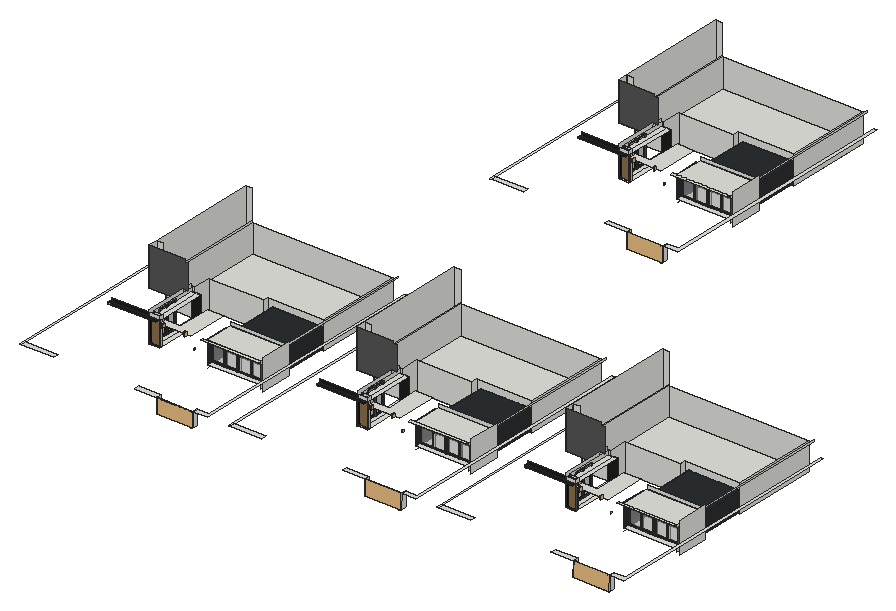
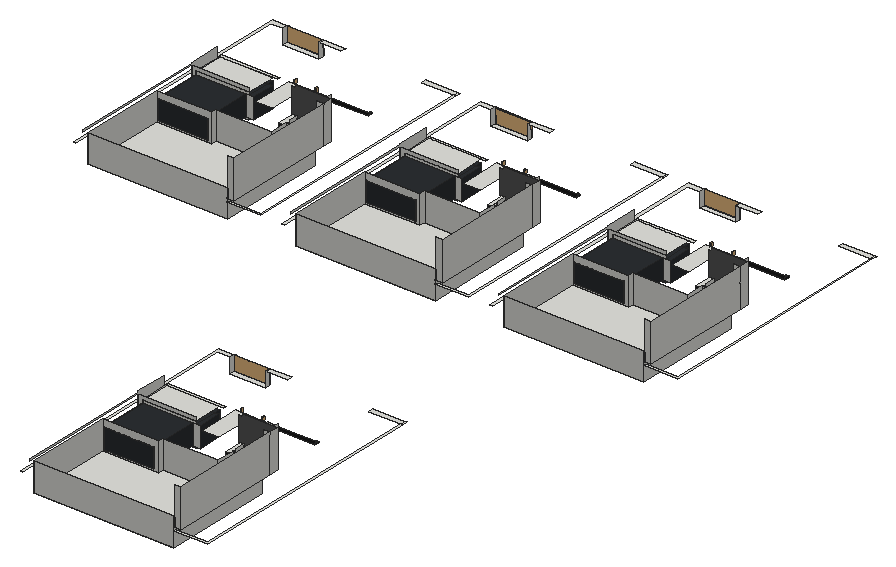
# SketchUp Ruby script. Lengths in inches.
U = 1.inch
M = Sketchup.active_model
def pt(a) = Geom::Point3d.new(a.map { |v| v * U })
def face(e, loops, mat)
  f = e.add_face(loops[0].map { |a| pt(a) })
  loops[1..].each { |l| e.add_face(l.map { |a| pt(a) }).erase! }
  f.material = f.back_material = mat if mat
  f
end
# faces: each face lists its corners as indices into pts; further lists are holes
def faces(e, pts, list, mat = nil) = list.each { |f| face(e, (f[0].is_a?(Array) ? f : [f]).map { |l| l.map { |i| pts[i] } }, mat) }
# xy, xz, yz: faces in a plane at the given z, y or x. An outline is a flat list of corners, or four numbers for a rectangle; further outlines are holes
def ring(l) = l.size == 4 ? [[l[0], l[1]], [l[2], l[1]], [l[2], l[3]], [l[0], l[3]]] : l.each_slice(2).to_a
def flat(e, list, mat, &to3) = list.each { |f| face(e, (f[0].is_a?(Array) ? f : [f]).map { |l| ring(l).map { |u, v| to3.(u, v) } }, mat) }
def xy(e, z, list, mat = nil) = flat(e, list, mat) { |x, y| [x, y, z] }
def xz(e, y, list, mat = nil) = flat(e, list, mat) { |x, z| [x, y, z] }
def yz(e, x, list, mat = nil) = flat(e, list, mat) { |y, z| [x, y, z] }
def lines(e, pts, list) = list.each { |a, b| e.add_line(pt(pts[a]), pt(pts[b])) }
# prism: a flat outline (further loops are holes) pulled along v
def prism(e, loops, v, mat = nil)
  f = face(e, loops, mat); d = Geom::Vector3d.new(v.map { |x| x * U })
  f.pushpull(f.normal.samedirection?(d) ? d.length : -d.length)
end
def box(e, o, s, mat = nil) = prism(e, [[o, [o[0] + s[0], o[1], o[2]], [o[0] + s[0], o[1] + s[1], o[2]], [o[0], o[1] + s[1], o[2]]]], [0, 0, s[2]], mat)
def at(x, y, z, deg = 0) = Geom::Transformation.translation(pt([x, y, z])) * Geom::Transformation.rotation(ORIGIN, Z_AXIS, deg.degrees)
def axes(o, x, y, z) = Geom::Transformation.new([*x, 0, *y, 0, *z, 0, *pt(o).to_a, 1])
def part(name) = M.definitions.add(name)
# library, detail: a bought-in or finely detailed component or shape, given as its bounding box
def library(name, o, s) = part(name).tap { |d| box(d.entities, o, s) }
def detail(e, o, s) = box(e.add_group.entities, o, s)
def put(e, d, t, mat = nil) = e.add_instance(d, t).tap { |i| i.material = mat if mat }
def group(e, t, mat = nil) = e.add_group.tap { |g| g.transformation = t; g.material = mat if mat }.entities
root = M.entities
M.materials.add("Antracyt").color = [44, 47, 50]
M.materials.add("Glass_Tinted_Gray").color = [0, 0, 0]
M.materials["Glass_Tinted_Gray"].alpha = 0.125
M.materials.add("[0135_DarkGray]").color = [81, 81, 81]
M.materials.add("[Color M00]").color = [255, 255, 255]
M.materials.add("[Color M04]").color = [60, 133, 34]
M.materials.add("[Color M06]1").color = [86, 86, 86]
M.materials.add("[Color M08]").color = [30, 30, 30]
M.materials.add("[Mirror 02]").color = [229, 229, 229]
M.materials.add("[Translucent Glass Gray]2").color = [201, 201, 201]
M.materials["[Translucent Glass Gray]2"].alpha = 0.5
M.materials.add("oak swatch").color = [40, 31, 19]
c1 = library("Group\#1",[0,0,0],[29.75,5.78,110.95])
c2 = part("PENTEK_RP Fineline 50S_SlidingDoor_Glass")
box(c2.entities,[0,0,0],[46.58,0.16,94.39],"Glass_Tinted_Gray")
c3 = part("PENTEK_RP Fineline 50S_SlidingDoor_GlazingBead")
box(c3.entities,[0,0,0],[45.47,0.59,0.56],"[0135_DarkGray]")
c4 = part("PENTEK_RP Fineline 50S_SlidingDoor_GlazingBead_2")
box(c4.entities,[0,0,0],[0.56,0.59,94.39],"[0135_DarkGray]")
c5 = part("PENTEK_RP Fineline 50S_SlidingDoor_Leaf_E1")
xy(c5.entities,0,[[0,0,0.93,1.97],[0.93,1.57,1.49,1.97]],"[0135_DarkGray]")
xy(c5.entities,96.25,[[0,0,0.93,0,0.93,1.57,1.49,1.57,1.49,1.97,0,1.97]],"[0135_DarkGray]")
xz(c5.entities,0,[[0,0,0.93,96.25]],"[0135_DarkGray]")
xz(c5.entities,1.57,[[0.93,0,1.49,95.32],[0.93,95.32,1.49,96.25]],"[0135_DarkGray]")
xz(c5.entities,1.97,[[0,0,1.49,96.25]],"[0135_DarkGray]")
yz(c5.entities,0,[[0,0,1.97,96.25]],"[0135_DarkGray]")
yz(c5.entities,0.93,[[0,0,1.57,0.93],[0,0.93,1.57,95.32],[0,95.32,1.57,96.25]],"[0135_DarkGray]")
yz(c5.entities,1.49,[[1.57,0,1.97,95.32],[1.57,95.32,1.97,96.25]],"[0135_DarkGray]")
c6 = part("PENTEK_RP Fineline 50S_SlidingDoor_Leaf_E2")
xy(c6.entities,0,[[0,0,0,1.57,0.56,1.57,0.56,1.97,46.02,1.97,46.02,1.57,46.58,1.57,46.58,0]],"[0135_DarkGray]")
xy(c6.entities,0.93,[[0,0,46.58,1.57]],"[0135_DarkGray]")
xy(c6.entities,1.49,[[0.56,1.57,46.02,1.97]],"[0135_DarkGray]")
xz(c6.entities,0,[[0,0,46.58,0.93]],"[0135_DarkGray]")
xz(c6.entities,1.57,[[0,0,0.56,0.93],[46.02,0,46.58,0.93],[0.56,0.93,46.02,1.49]],"[0135_DarkGray]")
xz(c6.entities,1.97,[[0.56,0,46.02,1.49]],"[0135_DarkGray]")
yz(c6.entities,0,[[0,0,1.57,0.93]],"[0135_DarkGray]")
yz(c6.entities,0.56,[[1.57,0,1.97,0.93],[1.57,0.93,1.97,1.49]],"[0135_DarkGray]")
yz(c6.entities,46.02,[[1.57,0,1.97,0.93],[1.57,0.93,1.97,1.49]],"[0135_DarkGray]")
yz(c6.entities,46.58,[[0,0,1.57,0.93]],"[0135_DarkGray]")
c7 = part("PENTEK_RP Fineline 50S_SlidingDoor_Leaf2")
put(c7.entities,c2,at(1.49,1.42,0.93))
put(c7.entities,c3,at(1.49,0,94.77))
put(c7.entities,c4,at(46.96,0,0.93))
put(c7.entities,c2,at(1.49,0.59,0.93),"[Mirror 02]")
put(c7.entities,c4,at(0.93,0,0.93))
put(c7.entities,c5,at(0,0,0))
put(c7.entities,c5,axes([48.44,0,0],[-1,0,0],[0,1,0],[0,0,1]))
put(c7.entities,c3,at(1.49,0,0.93))
put(c7.entities,c6,axes([0.93,0,96.25],[1,0,0],[0,1,0],[0,0,-1]))
put(c7.entities,c6,at(0.93,0,0))
c8 = library("1",[3.97,34.78,0],[101.43,33.99,0.79])
c9 = part("Group\#6")
box(c9.entities,[0,0,0],[1.77,4.72,80.31],"oak swatch")
c10 = part("Exterior Sliding Doors")
xy(c10.entities,0,[[1.77,33.07,3.54,70.87],[1.77,70.87,3.54,108.66]])
xy(c10.entities,0,[[0,0,1.77,33.07],[0,108.66,1.77,141.73]],"oak swatch")
xy(c10.entities,4.72,[[0,4.72,1.77,33.07],[1.77,37.8,3.54,66.14],[1.77,75.88,3.54,103.9375],[0,108.66,1.77,137.01]],"oak swatch")
xy(c10.entities,75.59,[[1.77,37.8,3.54,66.14],[1.77,75.88,3.54,103.9375]])
xy(c10.entities,75.59,[[0,4.72,1.77,33.07],[0,108.66,1.77,137.01]],"oak swatch")
xy(c10.entities,80.31,[[0,0,1.77,33.07],[1.77,33.07,3.54,70.87],[1.77,70.87,3.54,108.66],[0,108.66,1.77,141.73]],"oak swatch")
xz(c10.entities,0,[[0,0,1.77,80.31]],"oak swatch")
xz(c10.entities,4.72,[[0,4.72,1.77,75.59]],"oak swatch")
xz(c10.entities,33.07,[[0,0,1.77,4.72],[1.77,0,3.54,80.31],[0,75.59,1.77,80.31]],"oak swatch")
xz(c10.entities,37.8,[[1.77,4.72,3.54,75.59]])
xz(c10.entities,66.14,[[1.77,4.72,3.54,75.59]],"oak swatch")
xz(c10.entities,70.87,[[1.77,0,3.54,80.31]])
xz(c10.entities,75.88,[[1.77,4.72,3.54,75.59]])
xz(c10.entities,103.9375,[[1.77,4.72,3.54,75.59]],"oak swatch")
xz(c10.entities,108.66,[[1.77,4.72,3.54,75.59]])
xz(c10.entities,108.66,[[0,0,3.54,4.72],[0,75.59,3.54,80.31]],"oak swatch")
xz(c10.entities,137.01,[[0,4.72,1.77,75.59]],"oak swatch")
xz(c10.entities,141.73,[[0,0,1.77,80.31]],"oak swatch")
yz(c10.entities,0,[[0,0,33.07,0,33.07,4.72,4.72,4.72,4.72,75.59,33.07,75.59,33.07,80.31,0,80.31],[108.66,0,141.73,0,141.73,80.31,108.66,80.31,108.66,75.59,137.01,75.59,137.01,4.72,108.66,4.72]],"oak swatch")
yz(c10.entities,1.77,[[4.72,4.72,33.07,75.59],[37.8,4.72,66.14,75.59],[75.88,4.72,103.9375,75.59],[108.66,4.72,137.01,75.59]],"[Translucent Glass Gray]2")
yz(c10.entities,1.77,[[0,0,33.07,0,33.07,4.72,4.72,4.72,4.72,75.59,33.07,75.59,33.07,80.31,0,80.31],[[33.07,0,70.87,80.31],[37.8,4.72,66.14,75.59]],[[70.87,0,141.73,80.31],[108.66,4.72,137.01,75.59],[75.88,4.72,103.9375,75.59]]],"oak swatch")
yz(c10.entities,3.54,[[[33.07,0,70.87,80.31],[37.8,4.72,66.14,75.59]],[[70.87,0,108.66,80.31],[75.88,4.72,103.9375,75.59]]],"oak swatch")
put(c10.entities,c9,at(0,33.07,0))
put(c10.entities,c9,at(0,103.9375,0))
c11 = library("SPOT-EXTERIEUR",[0,-1.85,-3.93],[5.55,3.7,7.99])
c12 = library("Group\#13",[0,0,0],[3.54,3.54,3.9375])
xy(root,5.0625,[[424.39,505.3125,449.83,726.125],[449.83,505.3125,468.02,726.125],[1310.86,505.3125,1336.29,726.125],[1336.29,505.3125,1354.48,726.125],[2197.32,505.3125,2222.76,726.125],
  [2222.76,505.3125,2240.94,726.125],[312.24,732.16,435.61,732.16,435.61,807.47,671.5,807.47,671.5,829.91,908.11,829.91,908.11,1195.84,312.24,1195.84],[1198.7,732.16,1322.08,732.16,1322.08,807.47,1557.96,807.47,1557.96,829.91,1794.58,829.91,1794.58,1195.84,1198.7,1195.84],[2085.16,732.16,2208.54,732.16,2208.54,807.47,2444.43,807.47,2444.43,829.91,2681.04,829.91,2681.04,1195.84,2085.16,1195.84],[943.125,2357.31,968.5625,2578.12],
  [968.5625,2357.31,986.75,2578.12],[830.97,2584.15,954.34,2584.15,954.34,2659.46,1190.23,2659.46,1190.23,2681.9,1426.84,2681.9,1426.84,3047.84,830.97,3047.84]])
xy(root,9.9375,[[747.55,143.39,901.18,164.82],[1634.02,143.39,1787.65,164.82],[2520.48,143.39,2674.11,164.82],[1266.28,1995.38,1419.92,2016.82]])
xy(root,10.16,[[677.53,524.03,903.98,623.84],[1563.99,524.03,1790.45,623.84],[2450.46,524.03,2676.91,623.84],[1196.26,2376.02,1422.71,2475.84]])
xy(root,10.16,[[658.22,524.03,677.53,623.84],[1544.68,524.03,1563.99,623.84],[2431.15,524.03,2450.46,623.84],[690.86,623.84,903.98,829.91],[1577.32,623.84,1790.45,829.91],
  [2463.78,623.84,2676.91,829.91],[1176.95,2376.02,1196.26,2475.84],[1209.59,2475.84,1422.71,2681.9]],"Antracyt")
xy(root,18.41,[[677.53,498.6875,903.98,524.03],[1563.99,498.6875,1790.45,524.03],[2450.46,498.6875,2676.91,524.03],[1196.26,2350.68,1422.71,2376.02]])
xy(root,73,[[165.7,143.39,173.14,164.82],[173.14,143.39,308.39,164.82],[653.09,143.39,747.55,164.82],[901.18,143.39,962.46,143.39,962.46,1201.875,951.9375,1201.875,951.9375,164.82,901.18,164.82],[1052.17,143.39,1059.6,164.82],
  [1059.6,143.39,1194.85,164.82],[1539.55,143.39,1634.02,164.82],[1787.65,143.39,1848.92,143.39,1848.92,1201.875,1838.4,1201.875,1838.4,164.82,1787.65,164.82],[1938.63,143.39,1946.07,164.82],[1946.07,143.39,2081.32,164.82],
  [2426.02,143.39,2520.48,164.82],[2674.11,143.39,2735.38,143.39,2735.38,1201.875,2724.86,1201.875,2724.86,164.82,2674.11,164.82],[165.7,164.82,173.14,164.82,173.14,1192.15,310.02,1192.15,310.02,1201.875,165.7,1201.875],[1052.17,164.82,1059.6,164.82,1059.6,1192.15,1196.48,1192.15,1196.48,1201.875,1052.17,1201.875],[1938.63,164.82,1946.07,164.82,1946.07,1192.15,2082.95,1192.15,2082.95,1201.875,1938.63,1201.875],
  [684.43,1995.38,691.87,2016.82],[691.87,1995.38,827.12,2016.82],[1171.82,1995.38,1266.28,2016.82],[1419.92,1995.38,1481.1875,1995.38,1481.1875,3053.87,1470.67,3053.87,1470.67,2016.82,1419.92,2016.82],[684.43,2016.82,691.87,2016.82,691.87,3044.15,828.75,3044.15,828.75,3053.87,684.43,3053.87]])
xy(root,88,[[278.96,686.3125,424.39,726.125],[1165.42,686.3125,1310.86,726.125],[2051.88,686.3125,2197.32,726.125],[278.96,726.125,306.21,1201.875],[306.21,726.125,310.02,1201.875],
  [1165.42,726.125,1192.67,1201.875],[1192.67,726.125,1196.48,1201.875],[2051.88,726.125,2079.13,1201.875],[2079.13,726.125,2082.95,1201.875],[797.6875,2538.31,943.125,2578.12],
  [797.6875,2578.12,824.9375,3053.87],[824.9375,2578.12,828.75,3053.87]])
xy(root,97.03,[[677.53,498.6875,903.98,623.84],[1563.99,498.6875,1790.45,623.84],[2450.46,498.6875,2676.91,623.84],[658.22,524.03,677.53,623.84],[1544.68,524.03,1563.99,623.84],
  [2431.15,524.03,2450.46,623.84],[690.86,623.84,903.98,829.91],[1577.32,623.84,1790.45,829.91],[2463.78,623.84,2676.91,829.91],[1196.26,2350.68,1422.71,2475.84],
  [1176.95,2376.02,1196.26,2475.84],[1209.59,2475.84,1422.71,2681.9]],"Antracyt")
xy(root,110.1875,[[483.31,487.3125,483.31,521.5625,548.21,521.5625,548.21,662.5,618.43,662.5,618.43,487.3125],[658.22,487.3125,903.98,498.6875],[1369.77,487.3125,1369.77,521.5625,1434.68,521.5625,1434.68,662.5,1504.89,662.5,1504.89,487.3125],[1544.68,487.3125,1790.45,498.6875],[2256.23,487.3125,2256.23,521.5625,2321.14,521.5625,2321.14,662.5,2391.36,662.5,2391.36,487.3125],
  [2431.15,487.3125,2676.91,498.6875],[677.53,498.6875,903.98,623.84],[1563.99,498.6875,1790.45,623.84],[2450.46,498.6875,2676.91,623.84],[424.39,505.3125,435.61,521.5625],
  [435.61,505.3125,468.02,521.5625],[1310.86,505.3125,1322.08,521.5625],[1322.08,505.3125,1354.48,521.5625],[2197.32,505.3125,2208.54,521.5625],[2208.54,505.3125,2240.94,521.5625],
  [424.39,521.5625,429.58,726.125],[429.58,521.5625,449.83,726.125],[449.83,521.5625,468.02,726.125],[1310.86,521.5625,1316.04,726.125],[1316.04,521.5625,1336.29,726.125],
  [1336.29,521.5625,1354.48,726.125],[2197.32,521.5625,2202.51,726.125],[2202.51,521.5625,2222.76,726.125],[2222.76,521.5625,2240.94,726.125],[1002.04,2339.31,1002.04,2373.56,1066.94,2373.56,1066.94,2514.49,1137.16,2514.49,1137.16,2339.31],
  [1176.95,2339.31,1422.71,2350.68],[1196.26,2350.68,1422.71,2475.84],[943.125,2357.31,954.34,2373.56],[954.34,2357.31,986.75,2373.56],[943.125,2373.56,948.3125,2578.12],
  [948.3125,2373.56,968.5625,2578.12],[968.5625,2373.56,986.75,2578.12]])
xy(root,110.1875,[[264.14,487.3125,468.02,505.3125],[1150.61,487.3125,1354.48,505.3125],[2037.07,487.3125,2240.94,505.3125],[782.875,2339.31,986.75,2357.31]],"[Color M08]")
xz(root,487.3125,[[264.14,110.1875,270.875,115.91],[1150.61,110.1875,1157.34,115.91],[2037.07,110.1875,2043.8,115.91]])
xz(root,487.3125,[[270.875,110.1875,275.36,115.91],[1157.34,110.1875,1161.82,115.91],[2043.8,110.1875,2048.29,115.91]],"[Color M08]")
xz(root,505.3125,[[424.39,110.1875,468.02,125.0625],[1310.86,110.1875,1354.48,125.0625],[2197.32,110.1875,2240.94,125.0625]])
xz(root,505.3125,[[264.14,110.1875,424.39,125.0625],[1150.61,110.1875,1310.86,125.0625],[2037.07,110.1875,2197.32,125.0625]],"[Color M08]")
xz(root,521.5625,[[429.58,110.1875,435.61,125.0625],[435.61,110.1875,468.02,125.0625],[1316.04,110.1875,1322.08,125.0625],[1322.08,110.1875,1354.48,125.0625],[2202.51,110.1875,2208.54,125.0625],
  [2208.54,110.1875,2240.94,125.0625]])
xz(root,524.03,[[677.53,10.16,903.98,18.41],[1563.99,10.16,1790.45,18.41],[2450.46,10.16,2676.91,18.41]])
xz(root,524.03,[[658.22,10.16,677.53,97.03],[1544.68,10.16,1563.99,97.03],[2431.15,10.16,2450.46,97.03]],"Antracyt")
xz(root,623.84,[[677.53,5.0625,903.98,10.16],[903.98,5.0625,923.77,5.0625,923.77,125.0625,677.53,125.0625,677.53,110.1875,903.98,110.1875],[1563.99,5.0625,1790.45,10.16],[1790.45,5.0625,1810.23,5.0625,1810.23,125.0625,1563.99,125.0625,1563.99,110.1875,1790.45,110.1875],[2450.46,5.0625,2676.91,10.16],
  [2676.91,5.0625,2696.7,5.0625,2696.7,125.0625,2450.46,125.0625,2450.46,110.1875,2676.91,110.1875],[658.22,10.16,690.86,97.03],[1544.68,10.16,1577.32,97.03],[2431.15,10.16,2463.78,97.03],[677.53,97.03,903.98,110.1875],
  [1563.99,97.03,1790.45,110.1875],[2450.46,97.03,2676.91,110.1875]])
xz(root,686.3125,[[278.96,88,424.39,88,424.39,136.125,445.77,136.125,445.77,240.47,429.58,240.47,429.58,251.0625,278.96,251.0625],[1165.42,88,1310.86,88,1310.86,136.125,1332.23,136.125,1332.23,240.47,1316.04,240.47,1316.04,251.0625,1165.42,251.0625],[2051.88,88,2197.32,88,2197.32,136.125,2218.7,136.125,2218.7,240.47,2202.51,240.47,2202.51,251.0625,2051.88,251.0625]],"[Color M06]1")
xz(root,726.125,[[278.96,88,306.21,251.0625],[306.21,88,424.39,125.0625],[1165.42,88,1192.67,251.0625],[1192.67,88,1310.86,125.0625],[2051.88,88,2079.13,251.0625],
  [2079.13,88,2197.32,125.0625],[424.39,110.1875,429.58,125.0625],[1310.86,110.1875,1316.04,125.0625],[2197.32,110.1875,2202.51,125.0625]])
xz(root,726.125,[[429.58,5.0625,468.02,110.1875],[1316.04,5.0625,1354.48,110.1875],[2202.51,5.0625,2240.94,110.1875]],"[Color M08]")
xz(root,732.16,[[312.24,5.0625,435.61,125.0625],[1198.7,5.0625,1322.08,125.0625],[2085.16,5.0625,2208.54,125.0625]])
xz(root,807.47,[[435.61,5.0625,671.5,125.0625],[1322.08,5.0625,1557.96,125.0625],[2208.54,5.0625,2444.43,125.0625]])
xz(root,829.91,[[[671.5,5.0625,908.11,125.0625],[690.86,10.16,903.98,97.03]],[[1557.96,5.0625,1794.58,125.0625],[1577.32,10.16,1790.45,97.03]],[[2444.43,5.0625,2681.04,125.0625],[2463.78,10.16,2676.91,97.03]]])
xz(root,829.91,[[690.86,10.16,903.98,97.03],[1577.32,10.16,1790.45,97.03],[2463.78,10.16,2676.91,97.03]],"Antracyt")
xz(root,1195.84,[[312.24,5.0625,908.11,125.0625],[1198.7,5.0625,1794.58,125.0625],[2085.16,5.0625,2681.04,125.0625]])
xz(root,1201.875,[[278.96,88,306.21,251.0625],[1165.42,88,1192.67,251.0625],[2051.88,88,2079.13,251.0625]])
xz(root,2339.31,[[782.875,110.1875,789.61,115.91]])
xz(root,2339.31,[[789.61,110.1875,794.09,115.91]],"[Color M08]")
xz(root,2357.31,[[943.125,110.1875,986.75,125.0625]])
xz(root,2357.31,[[782.875,110.1875,943.125,125.0625]],"[Color M08]")
xz(root,2373.56,[[948.3125,110.1875,954.34,125.0625],[954.34,110.1875,986.75,125.0625]])
xz(root,2376.02,[[1196.26,10.16,1422.71,18.41]])
xz(root,2376.02,[[1176.95,10.16,1196.26,97.03]],"Antracyt")
xz(root,2475.84,[[1196.26,5.0625,1422.71,10.16],[1422.71,5.0625,1442.5,5.0625,1442.5,125.0625,1196.26,125.0625,1196.26,110.1875,1422.71,110.1875],[1176.95,10.16,1209.59,97.03],[1196.26,97.03,1422.71,110.1875]])
xz(root,2538.31,[[797.6875,88,943.125,88,943.125,136.125,964.5,136.125,964.5,240.47,948.3125,240.47,948.3125,251.0625,797.6875,251.0625]],"[Color M06]1")
xz(root,2578.12,[[797.6875,88,824.9375,251.0625],[824.9375,88,943.125,125.0625],[943.125,110.1875,948.3125,125.0625]])
xz(root,2578.12,[[948.3125,5.0625,986.75,110.1875]],"[Color M08]")
xz(root,2584.15,[[830.97,5.0625,954.34,125.0625]])
xz(root,2659.46,[[954.34,5.0625,1190.23,125.0625]])
xz(root,2681.9,[[[1190.23,5.0625,1426.84,125.0625],[1209.59,10.16,1422.71,97.03]]])
xz(root,2681.9,[[1209.59,10.16,1422.71,97.03]],"Antracyt")
xz(root,3047.84,[[830.97,5.0625,1426.84,125.0625]])
xz(root,3053.87,[[797.6875,88,824.9375,251.0625]])
yz(root,264.14,[[487.3125,110.1875,505.3125,115.66]],"[Color M08]")
yz(root,278.96,[[686.3125,88,726.125,251.0625],[726.125,88,1201.875,251.0625]])
yz(root,306.21,[[726.125,88,1201.875,125.0625]])
yz(root,312.24,[[732.16,5.0625,1195.84,125.0625]])
yz(root,424.39,[[686.3125,88,726.125,110.1875],[505.3125,110.1875,686.3125,136.125],[686.3125,110.1875,726.125,136.125]])
yz(root,429.58,[[521.5625,110.1875,726.125,125.0625]])
yz(root,435.61,[[732.16,5.0625,807.47,125.0625]])
yz(root,468.02,[[505.3125,110.1875,521.5625,125.0625]])
yz(root,658.22,[[524.03,10.16,623.84,97.03]],"Antracyt")
yz(root,671.5,[[807.47,5.0625,829.91,125.0625]])
yz(root,677.53,[[498.6875,18.41,524.03,97.03]],"Antracyt")
yz(root,690.86,[[623.84,10.16,829.91,97.03]],"Antracyt")
yz(root,747.55,[[143.39,9.9375,164.82,73]])
yz(root,782.875,[[2339.31,110.1875,2357.31,115.66]],"[Color M08]")
yz(root,797.6875,[[2538.31,88,2578.12,251.0625],[2578.12,88,3053.87,251.0625]])
yz(root,824.9375,[[2578.12,88,3053.87,125.0625]])
yz(root,830.97,[[2584.15,5.0625,3047.84,125.0625]])
yz(root,901.18,[[143.39,9.9375,164.82,73]])
yz(root,903.98,[[498.6875,5.0625,498.6875,18.41,524.03,18.41,524.03,10.16,623.84,10.16,623.84,5.0625],[498.6875,97.03,623.84,110.1875]])
yz(root,903.98,[[524.03,10.16,524.03,18.41,523.77,97.03,623.84,97.03,623.84,10.16],[623.84,10.16,829.91,97.03]],"Antracyt")
yz(root,903.98,[[523.77,18.41,523.77,97.03,524.03,18.41]],"[Color M00]")
yz(root,903.98,[[501.72,18.41,523.77,97.03]],"[Color M06]1")
yz(root,908.11,[[829.91,5.0625,1195.84,125.0625]])
yz(root,923.77,[[487.3125,5.0625,623.84,5.0625,623.84,125.0625,1201.875,125.0625,1201.875,131.0625,623.84,131.0625,623.84,136.125,487.3125,136.125]])
yz(root,943.125,[[2538.31,88,2578.12,110.1875],[2357.31,110.1875,2538.31,136.125],[2538.31,110.1875,2578.12,136.125]])
yz(root,948.3125,[[2373.56,110.1875,2578.12,125.0625]])
yz(root,954.34,[[2584.15,5.0625,2659.46,125.0625]])
yz(root,986.75,[[2357.31,110.1875,2373.56,125.0625]])
yz(root,1150.61,[[487.3125,110.1875,505.3125,115.66]],"[Color M08]")
yz(root,1165.42,[[686.3125,88,726.125,251.0625],[726.125,88,1201.875,251.0625]])
yz(root,1176.95,[[2376.02,10.16,2475.84,97.03]],"Antracyt")
yz(root,1190.23,[[2659.46,5.0625,2681.9,125.0625]])
yz(root,1192.67,[[726.125,88,1201.875,125.0625]])
yz(root,1196.26,[[2350.68,18.41,2376.02,97.03]],"Antracyt")
yz(root,1198.7,[[732.16,5.0625,1195.84,125.0625]])
yz(root,1209.59,[[2475.84,10.16,2681.9,97.03]],"Antracyt")
yz(root,1266.28,[[1995.38,9.9375,2016.82,73]])
yz(root,1310.86,[[686.3125,88,726.125,110.1875],[505.3125,110.1875,686.3125,136.125],[686.3125,110.1875,726.125,136.125]])
yz(root,1316.04,[[521.5625,110.1875,726.125,125.0625]])
yz(root,1322.08,[[732.16,5.0625,807.47,125.0625]])
yz(root,1354.48,[[505.3125,110.1875,521.5625,125.0625]])
yz(root,1419.92,[[1995.38,9.9375,2016.82,73]])
yz(root,1422.71,[[2350.68,5.0625,2350.68,18.41,2376.02,18.41,2376.02,10.16,2475.84,10.16,2475.84,5.0625],[2350.68,97.03,2475.84,110.1875]])
yz(root,1422.71,[[2376.02,10.16,2376.02,18.41,2375.77,97.03,2475.84,97.03,2475.84,10.16],[2475.84,10.16,2681.9,97.03]],"Antracyt")
yz(root,1422.71,[[2375.77,18.41,2375.77,97.03,2376.02,18.41]],"[Color M00]")
yz(root,1422.71,[[2353.71,18.41,2375.77,97.03]],"[Color M06]1")
yz(root,1426.84,[[2681.9,5.0625,3047.84,125.0625]])
yz(root,1442.5,[[2339.31,5.0625,2475.84,5.0625,2475.84,125.0625,3053.87,125.0625,3053.87,131.0625,2475.84,131.0625,2475.84,136.125,2339.31,136.125]])
yz(root,1544.68,[[524.03,10.16,623.84,97.03]],"Antracyt")
yz(root,1557.96,[[807.47,5.0625,829.91,125.0625]])
yz(root,1563.99,[[498.6875,18.41,524.03,97.03]],"Antracyt")
yz(root,1577.32,[[623.84,10.16,829.91,97.03]],"Antracyt")
yz(root,1634.02,[[143.39,9.9375,164.82,73]])
yz(root,1787.65,[[143.39,9.9375,164.82,73]])
yz(root,1790.45,[[498.6875,5.0625,498.6875,18.41,524.03,18.41,524.03,10.16,623.84,10.16,623.84,5.0625],[498.6875,97.03,623.84,110.1875]])
yz(root,1790.45,[[524.03,10.16,524.03,18.41,523.77,97.03,623.84,97.03,623.84,10.16],[623.84,10.16,829.91,97.03]],"Antracyt")
yz(root,1790.45,[[523.77,18.41,523.77,97.03,524.03,18.41]],"[Color M00]")
yz(root,1790.45,[[501.72,18.41,523.77,97.03]],"[Color M06]1")
yz(root,1794.58,[[829.91,5.0625,1195.84,125.0625]])
yz(root,1810.23,[[487.3125,5.0625,623.84,5.0625,623.84,125.0625,1201.875,125.0625,1201.875,131.0625,623.84,131.0625,623.84,136.125,487.3125,136.125]])
yz(root,2037.07,[[487.3125,110.1875,505.3125,115.66]],"[Color M08]")
yz(root,2051.88,[[686.3125,88,726.125,251.0625],[726.125,88,1201.875,251.0625]])
yz(root,2079.13,[[726.125,88,1201.875,125.0625]])
yz(root,2085.16,[[732.16,5.0625,1195.84,125.0625]])
yz(root,2197.32,[[686.3125,88,726.125,110.1875],[505.3125,110.1875,686.3125,136.125],[686.3125,110.1875,726.125,136.125]])
yz(root,2202.51,[[521.5625,110.1875,726.125,125.0625]])
yz(root,2208.54,[[732.16,5.0625,807.47,125.0625]])
yz(root,2240.94,[[505.3125,110.1875,521.5625,125.0625]])
yz(root,2431.15,[[524.03,10.16,623.84,97.03]],"Antracyt")
yz(root,2444.43,[[807.47,5.0625,829.91,125.0625]])
yz(root,2450.46,[[498.6875,18.41,524.03,97.03]],"Antracyt")
yz(root,2463.78,[[623.84,10.16,829.91,97.03]],"Antracyt")
yz(root,2520.48,[[143.39,9.9375,164.82,73]])
yz(root,2674.11,[[143.39,9.9375,164.82,73]])
yz(root,2676.91,[[498.6875,5.0625,498.6875,18.41,524.03,18.41,524.03,10.16,623.84,10.16,623.84,5.0625],[498.6875,97.03,623.84,110.1875]])
yz(root,2676.91,[[524.03,10.16,524.03,18.41,523.77,97.03,623.84,97.03,623.84,10.16],[623.84,10.16,829.91,97.03]],"Antracyt")
yz(root,2676.91,[[523.77,18.41,523.77,97.03,524.03,18.41]],"[Color M00]")
yz(root,2676.91,[[501.72,18.41,523.77,97.03]],"[Color M06]1")
yz(root,2681.04,[[829.91,5.0625,1195.84,125.0625]])
yz(root,2696.7,[[487.3125,5.0625,623.84,5.0625,623.84,125.0625,1201.875,125.0625,1201.875,131.0625,623.84,131.0625,623.84,136.125,487.3125,136.125]])
p = [[1563.99,623.84,5.0625],[1563.99,498.6875,5.0625],[2450.46,623.84,5.0625],[2450.46,498.6875,5.0625],[677.53,623.84,5.0625],[677.53,498.6875,5.0625],
  [1196.26,2475.84,5.0625],[1196.26,2350.68,5.0625]]
lines(root,p,[[0,1],[2,3],[4,5],[6,7]])
put(root,c1,axes([1310.86,514.94,1.68],[1.38276,0,0],[0,1,0],[0,0,1.03593]),"[Color M04]")
put(root,c1,axes([2197.32,514.94,1.68],[1.38276,0,0],[0,1,0],[0,0,1.03593]),"[Color M04]")
put(root,c1,axes([424.39,514.94,1.68],[1.38276,0,0],[0,1,0],[0,0,1.03593]),"[Color M04]")
put(root,c1,axes([943.125,2366.93,1.68],[1.38276,0,0],[0,1,0],[0,0,1.03593]),"[Color M04]")
put(root,c7,axes([1310.24,548.93,5.0625],[0,-0.90045,0],[1.1165,0,0],[0,0,1.08663]))
put(root,c7,axes([1310.86,592.56,5.0625],[0,-0.90045,0],[3.85,0,0],[0,0,1.1941]))
put(root,c7,axes([1310.86,506.89,5.0625],[0.90045,0,0],[0,1,0],[0,0,1.09216]))
put(root,c7,axes([1310.86,637.02,5.0625],[0,-0.90045,0],[3.85,0,0],[0,0,1.1941]))
put(root,c7,axes([2196.7,548.93,5.0625],[0,-0.90045,0],[1.1165,0,0],[0,0,1.08663]))
put(root,c7,axes([423.77,548.93,5.0625],[0,-0.90045,0],[1.1165,0,0],[0,0,1.08663]))
put(root,c7,axes([2197.32,592.56,5.0625],[0,-0.90045,0],[3.85,0,0],[0,0,1.1941]))
put(root,c7,axes([424.39,592.56,5.0625],[0,-0.90045,0],[3.85,0,0],[0,0,1.1941]))
put(root,c7,axes([2197.32,506.89,5.0625],[0.90045,0,0],[0,1,0],[0,0,1.09216]))
put(root,c7,axes([424.39,506.89,5.0625],[0.90045,0,0],[0,1,0],[0,0,1.09216]))
put(root,c7,axes([2197.32,637.02,5.0625],[0,-0.90045,0],[3.85,0,0],[0,0,1.1941]))
put(root,c7,axes([424.39,637.02,5.0625],[0,-0.90045,0],[3.85,0,0],[0,0,1.1941]))
put(root,c7,axes([943.125,2489.01,5.0625],[0,-0.90045,0],[3.85,0,0],[0,0,1.1941]))
put(root,c7,axes([943.125,2444.55,5.0625],[0,-0.90045,0],[3.85,0,0],[0,0,1.1941]))
put(root,c7,axes([942.51,2400.93,5.0625],[0,-0.90045,0],[1.1165,0,0],[0,0,1.08663]))
put(root,c7,axes([943.125,2358.88,5.0625],[0.90045,0,0],[0,1,0],[0,0,1.09216]))
put(root,c8,axes([1628,140.02,-53.07],[1.515,0,0],[0,0.06032,1.83265],[0,-1.49919,0.04935]))
put(root,c8,axes([2514.46,140.02,-53.07],[1.515,0,0],[0,0.06032,1.83265],[0,-1.49919,0.04935]))
put(root,c8,axes([741.53,140.02,-53.07],[1.515,0,0],[0,0.06032,1.83265],[0,-1.49919,0.04935]))
put(root,c8,axes([1260.26,1992.02,-53.07],[1.515,0,0],[0,0.06032,1.83265],[0,-1.49919,0.04935]))
put(root,c10,axes([1564.53,525.54,18.41],[0,-1,0],[1.59394,0,0],[0,0,0.97896]))
put(root,c10,axes([2451,525.54,18.41],[0,-1,0],[1.59394,0,0],[0,0,0.97896]))
put(root,c10,axes([678.07,525.54,18.41],[0,-1,0],[1.59394,0,0],[0,0,0.97896]))
put(root,c10,axes([1196.8,2377.54,18.41],[0,-1,0],[1.59394,0,0],[0,0,0.97896]))
put(root,c11,axes([1235.54,715.6875,58.23],[0,-0.68,0],[0.68,0,0],[0,0,0.68]))
put(root,c11,axes([2122,715.6875,58.23],[0,-0.68,0],[0.68,0,0],[0,0,0.68]))
put(root,c11,axes([349.08,715.6875,58.23],[0,-0.68,0],[0.68,0,0],[0,0,0.68]))
put(root,c11,axes([867.81,2567.68,58.23],[0,-0.68,0],[0.68,0,0],[0,0,0.68]))
put(root,c11,axes([1528.81,476.875,74.08],[0,-0.68,0],[0.68,0,0],[0,0,0.68]))
put(root,c11,axes([2415.27,476.875,74.08],[0,-0.68,0],[0.68,0,0],[0,0,0.68]))
put(root,c11,axes([642.35,476.875,74.08],[0,-0.68,0],[0.68,0,0],[0,0,0.68]))
put(root,c11,axes([1161.08,2328.87,74.08],[0,-0.68,0],[0.68,0,0],[0,0,0.68]))
put(root,c12,axes([1395.14,475.3125,121.92],[-1.5535,0,0],[0,2.39,0],[0,0,-3.63878]))
put(root,c12,axes([1486.76,475.3125,121.92],[-1.5535,0,0],[0,2.39,0],[0,0,-3.63878]))
put(root,c12,axes([2281.6,475.3125,121.92],[-1.5535,0,0],[0,2.39,0],[0,0,-3.63878]))
put(root,c12,axes([2373.23,475.3125,121.92],[-1.5535,0,0],[0,2.39,0],[0,0,-3.63878]))
put(root,c12,axes([508.68,475.3125,121.92],[-1.5535,0,0],[0,2.39,0],[0,0,-3.63878]))
put(root,c12,axes([600.3,475.3125,121.92],[-1.5535,0,0],[0,2.39,0],[0,0,-3.63878]))
put(root,c12,axes([1119.03,2327.31,121.92],[-1.5535,0,0],[0,2.39,0],[0,0,-3.63878]))
put(root,c12,axes([1027.41,2327.31,121.92],[-1.5535,0,0],[0,2.39,0],[0,0,-3.63878]))
